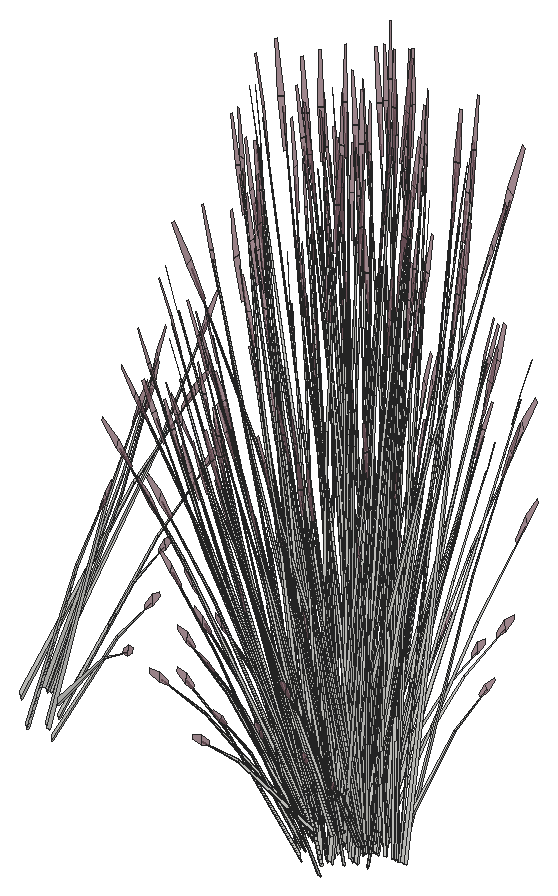
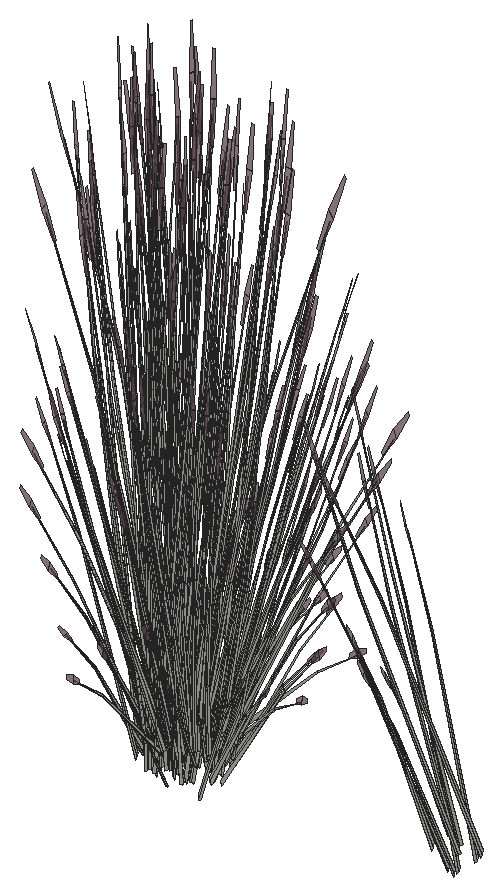
# SketchUp Ruby script. Lengths in inches.
U = 1.inch
M = Sketchup.active_model
def pt(a) = Geom::Point3d.new(a.map { |v| v * U })
def face(e, loops, mat)
  f = e.add_face(loops[0].map { |a| pt(a) })
  loops[1..].each { |l| e.add_face(l.map { |a| pt(a) }).erase! }
  f.material = f.back_material = mat if mat
  f
end
# faces: each face lists its corners as indices into pts; further lists are holes
def faces(e, pts, list, mat = nil) = list.each { |f| face(e, (f[0].is_a?(Array) ? f : [f]).map { |l| l.map { |i| pts[i] } }, mat) }
# xy, xz, yz: faces in a plane at the given z, y or x. An outline is a flat list of corners, or four numbers for a rectangle; further outlines are holes
def ring(l) = l.size == 4 ? [[l[0], l[1]], [l[2], l[1]], [l[2], l[3]], [l[0], l[3]]] : l.each_slice(2).to_a
def flat(e, list, mat, &to3) = list.each { |f| face(e, (f[0].is_a?(Array) ? f : [f]).map { |l| ring(l).map { |u, v| to3.(u, v) } }, mat) }
def xy(e, z, list, mat = nil) = flat(e, list, mat) { |x, y| [x, y, z] }
def xz(e, y, list, mat = nil) = flat(e, list, mat) { |x, z| [x, y, z] }
def yz(e, x, list, mat = nil) = flat(e, list, mat) { |y, z| [x, y, z] }
def lines(e, pts, list) = list.each { |a, b| e.add_line(pt(pts[a]), pt(pts[b])) }
# prism: a flat outline (further loops are holes) pulled along v
def prism(e, loops, v, mat = nil)
  f = face(e, loops, mat); d = Geom::Vector3d.new(v.map { |x| x * U })
  f.pushpull(f.normal.samedirection?(d) ? d.length : -d.length)
end
def box(e, o, s, mat = nil) = prism(e, [[o, [o[0] + s[0], o[1], o[2]], [o[0] + s[0], o[1] + s[1], o[2]], [o[0], o[1] + s[1], o[2]]]], [0, 0, s[2]], mat)
def at(x, y, z, deg = 0) = Geom::Transformation.translation(pt([x, y, z])) * Geom::Transformation.rotation(ORIGIN, Z_AXIS, deg.degrees)
def axes(o, x, y, z) = Geom::Transformation.new([*x, 0, *y, 0, *z, 0, *pt(o).to_a, 1])
def part(name) = M.definitions.add(name)
# library, detail: a bought-in or finely detailed component or shape, given as its bounding box
def library(name, o, s) = part(name).tap { |d| box(d.entities, o, s) }
def detail(e, o, s) = box(e.add_group.entities, o, s)
def put(e, d, t, mat = nil) = e.add_instance(d, t).tap { |i| i.material = mat if mat }
def group(e, t, mat = nil) = e.add_group.tap { |g| g.transformation = t; g.material = mat if mat }.entities
root = M.entities
M.materials.add("LightPink_Translucent").color = [144, 107, 117]
M.materials["LightPink_Translucent"].alpha = 0.75
c1 = part("blade")
p = [[2.15,0.21,22],[0,0.17,0],[0.09,0.45,0],[2.18,0.31,22],[2.29,0.31,22],[0.38,0.45,0],
  [2.48,0.24,33],[2.49,0.24,33],[2.48,0.22,33]]
faces(c1.entities,p,[[0,1,2,3],[4,5,2,3],[6,3,4,7],[8,0,3,6]])
c2 = part("seeds")
p = [[0.3,-0.1,1.38],[-0.01,-0.03,1.59],[-0.01,-0.03,0.03],[0.14,-0.07,-0.07],[0.29,-0.03,3],[0.15,0.01,3.11]]
faces(c2.entities,p,[[0,1,2,3],[1,0,4,5]],"LightPink_Translucent")
c3 = part("blade with seeds")
put(c3.entities,c1,at(0,0,0))
put(c3.entities,c2,axes([2.4,0.25,30.99],[1.5799,-0.05474,1.17369],[-0.12525,1.92788,0.29478],[-0.07173,-0.02425,1.56792]))
put(root,c3,axes([320.12,11.77,-3.41],[-0.27143,-0.0181,1.43002],[-0.27808,-0.48551,-0.30754],[0.33346,-0.13735,0.61141]))
put(root,c3,axes([320.3,13.48,-1.47],[0.63144,0.17046,-0.35414],[-0.18417,0.49731,0.4572],[0.25423,-0.0456,0.87481]))
put(root,c3,axes([319.08,14.55,-1.02],[0.75952,0.01471,-0.71045],[-0.05101,0.61953,0.08574],[0.32177,0.06538,1.00501]))
put(root,c3,axes([320.62,13.38,-4.02],[-0.48937,0.07333,1.41583],[-0.07789,-0.58369,0.08104],[0.34275,-0.08835,0.80566]))
put(root,c3,axes([321.15,13,-4.51],[-0.03971,-0.09277,1.76342],[0.27541,-0.54264,-0.26939],[0.27782,-0.00781,0.30037]))
put(root,c3,axes([321.42,15.34,-1.29],[-0.0687,-0.05349,1.77383],[0.15029,-0.57341,-0.16761],[0.27062,-0.03664,0.31391]))
put(root,c3,axes([318.58,12.86,-2.125],[-0.31515,0.01384,1.71376],[0.20907,-0.5998,0.13857],[0.44912,0.0371,0.73262]))
put(root,c3,axes([319.73,13.43,-1.02],[0.66765,-0.26986,-0.71045],[0.37208,0.55551,0.08574],[0.32259,-0.0631,1.00501]))
put(root,c3,axes([321.97,12.83,-1.28],[0.10543,-0.09307,1.74944],[-0.13495,-0.57092,-0.27667],[0.26455,-0.10825,0.14031]))
put(root,c3,axes([320.76,14.25,-3.41],[-0.18299,-0.15028,1.43002],[0.23809,-0.49714,-0.30754],[0.37023,0.06735,0.61141]))
put(root,c3,axes([344.33,12.17,-2.125],[0.31515,-0.01384,1.71376],[-0.20907,0.5998,0.13857],[-0.44912,-0.0371,0.73262]))
put(root,c3,axes([344.46,13.23,-2.125],[0.26363,-0.12925,1.71376],[0.22195,0.59723,0.13857],[-0.41388,0.13498,0.73262]))
put(root,c3,axes([343.64,14.24,-3.41],[0.26405,0.05016,1.43002],[0.17019,0.51235,-0.30754],[-0.35868,0.0959,0.61141]))
put(root,c3,axes([345.97,12.6,-2.66],[0.21597,-0.08839,1.77064],[0.07448,0.61717,0.13857],[-0.4678,0.08189,0.63284]))
put(root,c3,axes([343.65,13.02,-1.28],[-0.12407,0.07933,1.74944],[0.01055,0.57963,-0.27667],[-0.2844,0.07538,0.14031]))
put(root,c3,axes([345.27,11.61,-1.02],[-0.75952,-0.01471,-0.71045],[0.05101,-0.61953,0.08574],[-0.32177,-0.06538,1.00501]))
put(root,c3,axes([344.66,11.76,-3.41],[0.14835,0.17012,1.43002],[-0.34183,0.46242,-0.30754],[-0.351,-0.11053,0.61141]))
put(root,c3,axes([344.05,12.6875,-1.47],[-0.63144,-0.17046,-0.35414],[0.18417,-0.49731,0.4572],[-0.25423,0.0456,0.87481]))
put(root,c3,axes([344.92,11.21,-2.125],[0.28223,0.10528,1.71376],[-0.58406,0.44165,0.13857],[-0.36402,-0.19924,0.73262]))
put(root,c3,axes([342.27,13.6,-1.29],[0.09697,0.01639,1.77383],[0.29997,0.53988,-0.16761],[-0.1985,0.1417,0.31391]))
put(root,c3,axes([344.48,12.94,-1.32],[-0.20584,0.55581,-0.51099],[-0.70573,-0.19051,-0.3958],[-0.28414,0.05097,0.97773]))
put(root,c3,axes([345.02,11.74,-1.32],[-0.55171,0.40476,-0.51099],[-0.48318,-0.42758,-0.3958],[-0.28031,-0.06159,0.97773]))
put(root,c3,axes([344.13,12.91,-4.51],[0.01927,0.0963,1.76342],[-0.38846,0.5029,-0.26939],[-0.27592,-0.02535,0.30037]))
put(root,c3,axes([344.24,10.6,-1.29],[0.05633,0.06098,1.77383],[-0.27155,0.54815,-0.16761],[-0.27501,0.00397,0.31391]))
put(root,c3,axes([343.09,15.32,-3.23],[0.31665,-0.27694,1.1486],[0.12495,0.43841,0.84392],[-0.22883,0.0785,0.25299]))
put(root,c3,axes([344.87,10.24,-1.28],[-0.16348,-0.00431,1.74944],[-0.52047,0.43131,-0.27667],[-0.2777,-0.08813,0.14031]))
put(root,c3,axes([344.2,12.625,-1.27],[0.21466,-0.55714,0.48003],[0.70573,0.19051,0.3958],[-0.27753,0.03348,0.9933]))
put(root,c3,axes([344.45,12.46,-0.97],[0.38229,0.5533,-0.1216],[-0.6785,0.2719,-0.67495],[-0.28593,0.073,1.02557]))
put(root,c3,axes([345.31,11.32,-0.97],[-0.04068,0.62141,-0.1216],[-0.77029,-0.01698,-0.67495],[-0.29667,-0.04317,1.02557]))
put(root,c3,axes([344.81,11.36,-1.47],[-0.43232,-0.38257,-0.35414],[0.49364,-0.36215,0.4572],[-0.25081,-0.0551,0.87481]))
put(root,c3,axes([344.14,12.48,-1.27],[-0.27906,-0.41663,0.0643],[0.50888,-0.20393,0.50621],[-0.22432,0.04024,0.77189]))
put(root,c3,axes([345.42,13.63,-2.125],[0.18977,-0.18775,1.71376],[0.47917,0.50677,0.13857],[-0.32866,0.23079,0.73262]))
put(root,c3,axes([344.28,14.12,-1.47],[-0.66138,0.08733,-0.35414],[-0.17464,-0.49921,0.4572],[-0.18953,0.13408,0.87481]))
put(root,c3,axes([343.92,15.6,-4.51],[0.10192,0.06105,1.76342],[0.17281,0.56562,-0.26939],[-0.22588,0.12062,0.30037]))
put(root,c3,axes([343.78,12.28,-3.23],[0.48508,-0.04372,1.1486],[-0.3077,0.38525,0.84392],[-0.23971,-0.05779,0.25299]))
put(root,c3,axes([344.37,14.01,-1.27],[-0.18844,-0.56237,0.48003],[0.73919,-0.0976,0.3958],[-0.21785,0.13226,0.9933]))
put(root,c3,axes([344.75,11.21,-0.91],[0.62747,-0.45094,0.53763],[0.54116,0.47889,0.4433],[-0.29439,-0.08318,1.11249]))
put(root,c3,axes([344.22,13.9,-1.27],[-0.52161,-0.25698,0.0643],[0.30368,-0.36595,0.50621],[-0.16723,0.11831,0.77189]))
put(root,c3,axes([345.28,14.09,-2.125],[0.14147,-0.21002,1.71376],[0.59349,0.43464,0.13857],[-0.26773,0.27089,0.73262]))
put(root,c3,axes([344.72,12.63,-0.95],[0.63144,0.17046,0.35414],[-0.18417,0.49731,-0.4572],[-0.25423,0.0456,0.87481]))
put(root,c3,axes([344.83,14.18,-1.32],[0.19519,0.55794,-0.51099],[-0.73919,0.0976,-0.3958],[-0.21183,0.14986,0.97773]))
put(root,c3,axes([345.04,11.21,-1.27],[0.03826,-0.46465,0.0643],[0.57772,0.01274,0.50621],[-0.2213,-0.04862,0.77189]))
put(root,c3,axes([343.67,15.18,-1.28],[-0.01889,0.12092,1.74944],[0.53598,0.42065,-0.27667],[-0.14032,0.19892,0.14031]))
put(root,c3,axes([346.67,13.78,-3.94],[-0.79037,-0.10018,-0.62353],[0.16679,-0.61794,-0.16365],[-0.23587,-0.07488,1.37633]))
put(root,c3,axes([346.8125,10.41,-0.57],[-0.50709,0.58578,-0.13619],[-0.73436,-0.33748,-0.75594],[-0.25527,-0.1655,1.14864]))
put(root,c3,axes([345.43,11.56,-0.95],[0.43232,0.38257,0.35414],[-0.49364,0.36215,-0.4572],[-0.25081,-0.0551,0.87481]))
put(root,c3,axes([346.59,10.88,-1.02],[-0.64788,-0.29534,-0.71045],[0.46044,-0.51755,0.08574],[-0.23473,-0.17635,1.00501]))
put(root,c3,axes([346.29,10.9,-1.32],[-0.74975,0.14525,-0.51099],[-0.13115,-0.55007,-0.3958],[-0.20138,-0.15763,0.97773]))
put(root,c3,axes([345.63,14.95,-3.98],[-0.7111,-0.30552,-0.49651],[0.42504,-0.54784,0],[-0.16196,-0.06958,1.57504]))
put(root,c3,axes([345.32,10.4,-4.51],[-0.0736,0.08049,1.76342],[-0.74378,0.17355,-0.26939],[-0.17968,-0.15788,0.30037]))
put(root,c3,axes([344.48,13.78,-0.97],[0.70283,0.33692,-0.1216],[-0.40491,0.48793,-0.67495],[-0.19857,0.16961,1.02557]))
put(root,c3,axes([346.07,15.32,-3.625],[-0.47504,0.61229,0],[-0.79476,-0.34146,-0.51607],[-0.18101,-0.07777,1.63711]))
put(root,c3,axes([343.32,15.24,-0.35],[0.67048,0.16311,-0.06488],[-0.20625,0.50201,-0.29416],[-0.10966,0.07622,0.97024]))
put(root,c3,axes([344.82,13.83,-0.95],[0.66138,-0.08733,0.35414],[0.17464,0.49921,-0.4572],[-0.18953,0.13408,0.87481]))
put(root,c3,axes([345.2,16.2,-3.41],[0.23977,-0.09639,1.43002],[0.59198,0.29065,-0.30754],[-0.1762,0.25149,0.61141]))
put(root,c3,axes([344.86,10.71,-3.87],[-0.21918,0.49894,-0.03893],[-0.6746,-0.15348,-0.17649],[-0.10242,-0.08161,0.58215]))
put(root,c3,axes([346.62,9.02,-1.29],[-0.01417,0.07324,1.77383],[-0.6991,0.2658,-0.16761],[-0.20573,-0.13587,0.31391]))
put(root,c3,axes([345.87,10.08,-3.41],[-0.04601,0.19989,1.43002],[-0.67263,0.16733,-0.30754],[-0.15723,-0.25836,0.61141]))
put(root,c3,axes([346.09,10.6,-2.125],[0.17368,0.19618,1.71376],[-0.80256,0.16516,0.13857],[-0.18139,-0.30799,0.73262]))
put(root,c3,axes([347.57,13.87,-3.33],[-0.76714,0.40567,-0.29095],[-0.51013,-0.57321,-0.50002],[-0.18927,-0.05821,1.59708]))
put(root,c3,axes([345.45,15.15,-1.27],[-0.54105,-0.41691,0.48003],[0.57458,-0.35956,0.3958],[-0.0998,0.1956,0.9933]))
put(root,c3,axes([346.37,10.49,-1.47],[-0.11735,-0.49217,-0.35414],[0.67083,-0.12996,0.4572],[-0.18018,-0.14104,0.87481]))
put(root,c3,axes([344.5,12.99,-3.625],[-0.95008,0,0],[0,-0.68292,-0.51607],[0,-0.15554,1.63711]))
put(root,c3,axes([345.83,14.72,-3.97],[-0.17848,-0.53243,-0.30978],[0.70886,-0.15119,0.30978],[-0.1429,-0.0614,1.38974]))
put(root,c3,axes([345.25,15.11,-1.27],[-0.62439,-0.02847,0.0643],[0.01712,-0.42991,0.50621],[-0.06534,0.16468,0.77189]))
put(root,c3,axes([345.45,15.28,-1.47],[-0.5141,0.32171,-0.35414],[-0.48666,-0.36734,0.4572],[-0.07405,0.18664,0.87481]))
put(root,c3,axes([348.08,14.3125,-3.94],[-0.51177,0.45928,-0.62353],[-0.63575,-0.41646,-0.16365],[-0.20507,0.11457,1.37633]))
put(root,c3,axes([346.76,10.89,-0.95],[0.11735,0.49217,0.35414],[-0.67083,0.12996,-0.4572],[-0.18018,-0.14104,0.87481]))
put(root,c3,axes([343.61,16.42,-1.29],[0.0862,-0.03689,1.77383],[0.71245,0.24539,-0.16761],[-0.01674,0.20431,0.31391]))
put(root,c3,axes([345.23,12.81,-3.67],[-0.70674,0.51372,0.30756],[-0.70717,-0.50832,-0.36492],[-0.02468,-0.14589,1.64885]))
put(root,c3,axes([348.14,14.22,-2.67],[0.65659,0.2464,1.51261],[-0.64324,0.53082,0.59816],[-0.28812,-0.31461,1.26806]))
put(root,c3,axes([345.64,9.76,-3.23],[0.39634,0.21267,1.1486],[-0.57721,0.12784,0.84392],[-0.1235,-0.16344,0.25299]))
put(root,c3,axes([348.43,14.05,-3.54],[-0.74193,-0.49181,-0.25192],[0.6243,-0.55226,0.5513],[-0.19979,0.05753,1.68216]))
put(root,c3,axes([347.08,13.58,-3.79],[-0.45644,-0.51287,-0.44739],[0.69137,-0.36116,0.21531],[-0.14771,-0.06346,1.43643]))
put(root,c3,axes([345.79,14.9375,-0.66],[-0.01977,0.56521,-0.7886],[-0.83252,-0.03796,0.09517],[-0.08786,0.23945,1.11556]))
put(root,c3,axes([345.77,16.53,-3.23],[-0.01966,-0.36332,1.1486],[0.49135,0.25914,0.84392],[-0.09663,0.17317,0.25299]))
put(root,c3,axes([346.46,10.31,-0.91],[0.84639,-0.15705,0.53763],[0.14689,0.61608,0.4433],[-0.19906,-0.18157,1.11249]))
put(root,c3,axes([348.05,13.95,-3.79],[-0.82508,0.03772,-0.44739],[-0.07462,-0.62614,0.21531],[-0.14771,0.06346,1.43643]))
put(root,c3,axes([346.66,10.45,-1.27],[0.34533,-0.38816,0.0643],[0.49176,0.22599,0.50621],[-0.15898,-0.12445,0.77189]))
put(root,c3,axes([346.48,15,-3.52],[0.7111,0.30552,0.49651],[-0.42504,0.54784,0],[-0.16196,-0.06958,1.57504]))
put(root,c3,axes([345.51,15.73,-2.64],[0.01669,-0.31544,1.54345],[0.75083,0.16661,0.21329],[-0.06506,0.33618,0.72882]))
put(root,c3,axes([347.15,13.875,-3.5625],[0.20138,-0.72405,-0.23429],[0.95485,0.12621,0.51271],[-0.16685,-0.09999,1.5644]))
put(root,c3,axes([347.49,14.05,-3.38],[-0.14658,0.54532,0.1448],[-0.71613,-0.09466,-0.41347],[-0.13033,-0.05599,1.26744]))
put(root,c3,axes([347.41,9.3,-1.28],[-0.11621,-0.08567,1.74944],[-0.77555,0.05431,-0.27667],[-0.12378,-0.20491,0.14031]))
put(root,c3,axes([348.92,15.57,-3.98],[-0.7111,0.30552,-0.49651],[-0.42504,-0.54784,0],[-0.16196,0.06958,1.57504]))
put(root,c3,axes([344.71,12.52,-3.98],[0,-0.61104,-0.49651],[0.85008,0,0],[0,-0.13917,1.57504]))
put(root,c3,axes([345.07,13.09,-3.52],[0,0.61104,0.49651],[-0.85008,0,0],[0,-0.13917,1.57504]))
put(root,c3,axes([348.97,15.4,-3.81],[-0.46912,-0.61443,-0.05142],[0.79476,-0.34146,0.51607],[-0.19584,0.0585,1.6363]))
put(root,c3,axes([345.96,15.125,-1],[0.54391,0.41056,-0.5672],[-0.57458,0.35956,-0.43934],[-0.08276,0.2086,1.08528]))
put(root,c3,axes([348.75,15.32,-3.97],[-0.70886,-0.15119,-0.30978],[0.17848,-0.53243,0.30978],[-0.1429,0.0614,1.38974]))
put(root,c3,axes([345.71,14.82,-0.95],[0.5141,-0.32171,0.35414],[0.48666,0.36734,-0.4572],[-0.07405,0.18664,0.87481]))
put(root,c3,axes([346.93,13.23,-3.33],[-0.85568,-0.29155,-0.29095],[0.41201,-0.61537,-0.50002],[-0.02689,-0.15109,1.59708]))
put(root,c3,axes([349.16,13.05,-3.16],[-0.02076,-0.57531,1.41272],[0.93937,0.14913,0.59816],[-0.22217,0.31481,1.3335]))
put(root,c3,axes([345.39,14.91,-0.6],[0.83505,0.03027,-0.13498],[-0.02282,0.57322,-0.74919],[-0.05801,0.22077,1.13838]))
put(root,c3,axes([345.37,15.74,-3.18],[0.69024,-0.1082,0.06507],[0.15868,0.43593,-0.86304],[-0.04376,0.22067,0.7736]))
put(root,c3,axes([348.63,13.78,-3.33],[0.08854,0.69723,-0.29095],[-0.92215,0.04216,-0.50002],[-0.16238,0.09287,1.59708]))
put(root,c3,axes([346.55,12.61,-3.9],[-0.31203,-0.62659,-0.69835],[0.89884,-0.22566,-0.18329],[-0.03449,-0.21218,1.54149]))
put(root,c3,axes([348.59,10.62,-0.97],[-0.74352,0.28449,-0.1216],[-0.36538,-0.50492,-0.67495],[-0.0981,-0.21277,1.02557]))
put(root,c3,axes([347.95,10.64,-1.32],[-0.7469,-0.15318,-0.51099],[0.25601,-0.52518,-0.3958],[-0.06849,-0.21144,0.97773]))
put(root,c3,axes([346.58,14.54,-2.125],[-0.0186,-0.23452,1.71376],[0.80601,0.15558,0.13857],[-0.04985,0.33422,0.73262]))
put(root,c3,axes([345.07,12.54,-3.97],[0.53038,-0.38124,-0.30978],[0.53038,0.38124,0.30978],[0,-0.1228,1.38974]))
put(root,c3,axes([347.47,10.07,-3.87],[-0.52505,0.35054,-0.03893],[-0.48109,-0.38392,-0.17649],[-0.03387,-0.10878,0.58215]))
put(root,c3,axes([347.26,13.53,-3.64],[0.96033,0.12874,0.45755],[-0.19544,0.7271,0.17955],[-0.14034,-0.07021,1.58856]))
put(root,c3,axes([347.01,13.4,-3.28],[-0.36864,0.55059,0.44739],[-0.76598,-0.26498,-0.21531],[0,-0.12692,1.43643]))
put(root,c3,axes([348.23,10.74,-1.02],[-0.36264,-0.49684,-0.71045],[0.74649,-0.27689,0.08574],[-0.0848,-0.24006,1.00501]))
put(root,c3,axes([346.74,14.6875,-3.53],[0.81646,-0.16218,0.17642],[0.20161,0.60355,0.35086],[-0.07282,-0.08794,1.60407]))
put(root,c3,axes([347.79,14.78,-3.8],[-0.76598,-0.27433,0],[0.36864,-0.57001,0],[0,0,1.62707]))
put(root,c3,axes([348.37,10.82,-0.95],[-0.22906,0.4699,0.35414],[-0.66828,-0.13705,-0.4572],[-0.06128,-0.18919,0.87481]))
put(root,c3,axes([349.57,15.47,-3.625],[0.47504,0.61229,0],[-0.79476,0.34146,-0.51607],[-0.18101,0.07777,1.63711]))
put(root,c3,axes([347.15,15.73,-0.9375],[-0.74868,-0.15974,0.53283],[0.25601,-0.52518,0.43934],[0.04499,0.20653,1.10256]))
put(root,c3,axes([346.95,15.77,-1.27],[-0.55987,0.20767,0.0643],[-0.27403,-0.37869,0.50621],[0.05407,0.16693,0.77189]))
put(root,c3,axes([349.17,14.72,-3.53],[0.21949,-0.60727,0.17642],[0.8032,0.17185,0.35086],[-0.13875,0.00296,1.60407]))
put(root,c3,axes([348.8,13.92,-3.38],[0.56134,0.36712,0.1448],[-0.46823,0.41419,-0.41347],[-0.13033,0.05599,1.26744]))
put(root,c3,axes([348.6,13.46,-3.7],[-0.70674,-0.52593,-0.06131],[0.70717,-0.52625,0],[-0.02468,-0.01837,1.75571]))
put(root,c3,axes([348.79,13.65,-3.28],[0.82508,-0.03772,0.44739],[0.07462,0.62614,-0.21531],[-0.14771,0.06346,1.43643]))
put(root,c3,axes([348.99,15.09,-3.67],[0.95122,0.19861,0.30756],[-0.23797,0.7099,-0.36492],[-0.15744,0.08885,1.64885]))
put(root,c3,axes([347.6,9.64,-4.51],[-0.12744,0.02202,1.76342],[-0.70477,-0.24781,-0.26939],[0.01183,-0.2067,0.30037]))
put(root,c3,axes([349.4,15.05,-3.52],[0.7111,-0.30552,0.49651],[0.42504,0.54784,0],[-0.16196,0.06958,1.57504]))
put(root,c3,axes([348.29,10.32,-1.47],[0.22906,-0.4699,-0.35414],[0.66828,0.13705,0.4572],[-0.06128,-0.18919,0.87481]))
put(root,c3,axes([347.18,12.86,-3.64],[0.33034,0.68327,0.45755],[-0.94388,0.2376,0.17955],[0.01154,-0.12555,1.58856]))
put(root,c3,axes([347.02,12.77,-3.79],[0.36864,-0.55059,-0.44739],[0.76598,0.26498,0.21531],[0,-0.12692,1.43643]))
put(root,c3,axes([347.97,14.55,-3.8],[-0.24791,-0.5268,0],[0.70791,-0.18448,0],[0,0,1.54371]))
put(root,c3,axes([347.07,15.66,-4.51],[0.12297,-0.03325,1.76342],[0.73967,0.18301,-0.26939],[0.02163,0.20626,0.30037]))
put(root,c3,axes([347.23,15.84,-1.47],[-0.22906,0.4699,-0.35414],[-0.66828,-0.13705,0.4572],[0.06128,0.18919,0.87481]))
put(root,c3,axes([348.97,13.51,-3.79],[-0.36864,0.55059,-0.44739],[-0.76598,-0.26498,0.21531],[0,0.12692,1.43643]))
put(root,c3,axes([348.58,10.39,-1.27],[0.55987,-0.20767,0.0643],[0.27403,0.37869,0.50621],[-0.05407,-0.16693,0.77189]))
put(root,c3,axes([346.76,16.68,-1.28],[0.09631,0.0984,1.74944],[0.77725,0.03866,-0.27667],[0.07816,0.217,0.14031]))
put(root,c3,axes([350.43,13.17,-3.53],[-0.59697,-0.44509,0.17642],[0.60159,-0.4317,0.35086],[-0.06593,0.0909,1.60407]))
put(root,c3,axes([348.36,12.92,-3.79],[0,-0.70701,0],[0.95008,0,0],[0,0,1.79456]))
put(root,c3,axes([348.38,10.43,-1.27],[0.74868,0.15974,0.48003],[-0.25601,0.52518,0.3958],[-0.04499,-0.20653,0.9933]))
put(root,c3,axes([347.48,13.04,-3.57],[0.8561,0.29616,0.24065],[-0.41201,0.61537,0.50002],[0,-0.14185,1.60543]))
put(root,c3,axes([348.84,13.2,-3.71],[0,0.70667,-0.05637],[-0.95008,0,0],[0,0.02221,1.79368]))
put(root,c3,axes([347.2,12.63,-3.28],[-0.82508,0.03772,0.44739],[-0.07462,-0.62614,-0.21531],[0.14771,-0.06346,1.43643]))
put(root,c3,axes([347.16,15.35,-0.95],[0.22906,-0.4699,0.35414],[0.66828,0.13705,-0.4572],[0.06128,0.18919,0.87481]))
put(root,c3,axes([346.82,11.56,-3.53],[-0.21949,0.60727,0.17642],[-0.8032,-0.17185,0.35086],[0.13875,-0.00296,1.60407]))
put(root,c3,axes([348.39,14.57,-3.71],[0.33034,0.70197,-0.06012],[-0.94388,0.24598,0],[0.01154,0.02451,1.72173]))
put(root,c3,axes([346.43,10.81,-3.625],[-0.47504,-0.61229,0],[0.79476,-0.34146,-0.51607],[0.18101,-0.07777,1.63711]))
put(root,c3,axes([347.3,15.42,-1.02],[0.36264,0.49684,-0.71045],[-0.74649,0.27689,0.08574],[0.0848,0.24006,1.00501]))
put(root,c3,axes([351.11,13.64,-3.8],[-0.94962,-0.00489,-0.04976],[0,-0.68292,0.49943],[-0.02984,0.15546,1.58352]))
put(root,c3,axes([349.25,11.59,-3.53],[-0.81646,0.16218,0.17642],[-0.20161,-0.60355,0.35086],[0.07282,0.08794,1.60407]))
put(root,c3,axes([348.42,9.33,-3.23],[0.09747,0.35631,1.1486],[-0.54071,-0.19735,0.84392],[0.05818,-0.18244,0.25299]))
put(root,c3,axes([348.06,17.03,-0.35],[0.52505,-0.35054,-0.06488],[0.48109,0.38392,-0.29416],[0.03387,0.10878,0.97024]))
put(root,c3,axes([347.91,12.47,-3.64],[-0.62999,0.55453,0.45755],[-0.74845,-0.4895,0.17955],[0.15188,-0.05534,1.58856]))
put(root,c3,axes([348.99,13.34,-3.79],[0.53038,0.39469,0],[-0.53038,0.39469,0],[0,0,1.69266]))
put(root,c3,axes([348.98,12.88,-3.28],[0.36864,-0.55059,0.44739],[0.76598,0.26498,-0.21531],[0,0.12692,1.43643]))
put(root,c3,axes([348.66,14.8,-3.8],[0.76598,0.27433,0],[-0.36864,0.57001,0],[0,0,1.74954]))
put(root,c3,axes([347.57,15.52,-1.32],[0.7469,0.15318,-0.51099],[-0.25601,0.52518,-0.3958],[0.06849,0.21144,0.97773]))
put(root,c3,axes([346.93,15.55,-0.97],[0.74352,-0.28449,-0.1216],[0.36538,0.50492,-0.67495],[0.0981,0.21277,1.02557]))
put(root,c3,axes([348.73,12.75,-3.62],[-0.96033,-0.12874,0.49198],[0.19544,-0.7271,0.19306],[0.14034,0.07021,1.70813]))
put(root,c3,axes([350.73,9.91,-1.29],[-0.07716,0.04667,1.77383],[-0.75601,-0.15746,-0.16761],[-0.02737,-0.20368,0.31391]))
put(root,c3,axes([350.14,11.26,-0.97],[-0.83505,-0.03027,-0.1216],[0.02282,-0.57322,-0.67495],[0.05801,-0.22077,1.02557]))
put(root,c3,axes([350.92,13.74,-3.97],[-0.53038,0.38124,-0.30978],[-0.53038,-0.38124,0.30978],[0,0.1228,1.38974]))
put(root,c3,axes([349.4,13.67,-3.91],[0.2786,0.55945,-0.69212],[-0.80253,0.20149,-0.18165],[0.03079,0.18945,1.52773]))
put(root,c3,axes([349.01,13.07,-3.79],[0.85008,0,0],[0,0.63259,0],[0,0,1.78407]))
put(root,c3,axes([349.81,11.35,-0.95],[-0.5141,0.32171,0.35414],[-0.48666,-0.36734,-0.4572],[0.07405,-0.18664,0.87481]))
put(root,c3,axes([348.19,12.375,-3.28],[-0.45644,-0.51287,0.44739],[0.69137,-0.36116,-0.21531],[0.14771,0.06346,1.43643]))
put(root,c3,axes([347.36,12.5,-3.33],[-0.08854,-0.69723,-0.29095],[0.92215,-0.04216,-0.50002],[0.16238,-0.09287,1.59708]))
put(root,c3,axes([349.3,13.01,-3.38],[0.70791,-0.1782,0.1448],[0.24791,0.50885,-0.41347],[0,0.11199,1.26744]))
put(root,c3,axes([349.57,11.04,-1.32],[-0.54391,-0.41056,-0.51099],[0.57458,-0.35956,-0.3958],[0.08276,-0.2086,0.97773]))
put(root,c3,axes([349.06,13.05,-3.33],[0.85568,0.29155,-0.29095],[-0.41201,0.61537,-0.50002],[0.02689,0.15109,1.59708]))
put(root,c3,axes([347.24,10.95,-3.97],[0.70886,0.15119,-0.30978],[-0.17848,0.53243,0.30978],[0.1429,-0.0614,1.38974]))
put(root,c3,axes([349.21,10.3125,-3.41],[-0.21597,0.12368,1.43002],[-0.64681,-0.21647,-0.30754],[0.1199,-0.26922,0.61141]))
put(root,c3,axes([350.92,13.19,-3.52],[0,-0.61104,0.49651],[0.85008,0,0],[0,0.13917,1.57504]))
put(root,c3,axes([351.28,13.76,-3.98],[0,0.61104,-0.49651],[-0.85008,0,0],[0,0.13917,1.57504]))
put(root,c3,axes([349.01,15.61,-1.27],[-0.75571,0.14023,0.48003],[-0.13115,-0.55007,0.3958],[0.17773,0.16212,0.9933]))
put(root,c3,axes([347.07,10.71,-3.98],[0.7111,-0.30552,-0.49651],[0.42504,0.54784,0],[0.16196,-0.06958,1.57504]))
put(root,c3,axes([348.87,15.72,-1.27],[-0.34533,0.38816,0.0643],[-0.49176,-0.22599,0.50621],[0.15898,0.12445,0.77189]))
put(root,c3,axes([347.99,14.4375,-2.125],[-0.17368,-0.19618,1.71376],[0.80256,-0.16516,0.13857],[0.18139,0.30799,0.73262]))
put(root,c3,axes([348.5,12.23,-3.38],[0.14658,-0.54532,0.1448],[0.71613,0.09466,-0.41347],[0.13033,0.05599,1.26744]))
put(root,c3,axes([349.52,11.28,-3.52],[-0.7111,-0.30552,0.49651],[0.42504,-0.54784,0],[0.16196,0.06958,1.57504]))
put(root,c3,axes([349.74,11.23,-1.02],[0.01977,-0.56521,-0.71045],[0.83252,0.03796,0.08574],[0.08786,-0.23945,1.00501]))
put(root,c3,axes([348.9,14.47,-3.82],[0.79769,-0.20732,-0.19198],[0.2803,0.59721,0.00008],[0.08805,-0.02292,1.73897]))
put(root,c3,axes([348.76,15.27,-0.95],[-0.11735,-0.49217,0.35414],[0.67083,-0.12996,-0.4572],[0.18018,0.14104,0.87481]))
put(root,c3,axes([348.91,12.7,-3.79],[0.45644,0.51287,-0.44739],[-0.69137,0.36116,0.21531],[0.14771,0.06346,1.43643]))
put(root,c3,axes([349.21,12.44,-1.53],[-0.65655,-0.31748,1.38283],[0.69326,-0.49431,0.59665],[0.21183,0.29789,1.33663]))
put(root,c3,axes([350.08,10.89,-1.47],[0.5141,-0.32171,-0.35414],[0.48666,0.36734,0.4572],[0.07405,-0.18664,0.87481]))
put(root,c3,axes([348.11,15.96,-1.29],[0.00225,-0.07398,1.77383],[0.65113,-0.32638,-0.16761],[0.22617,0.1165,0.31391]))
put(root,c3,axes([350.28,11.05,-1.27],[0.62439,0.02847,0.0643],[-0.01712,0.42991,0.50621],[0.06534,-0.16468,0.77189]))
put(root,c3,axes([350.2,15.02,-3.23],[-0.4278,-0.1757,1.1486],[0.5524,-0.17852,0.84392],[0.14899,0.15122,0.25299]))
put(root,c3,axes([348.68,14.84,-3.41],[0.01341,-0.20255,1.43002],[0.64074,-0.22625,-0.30754],[0.1978,0.24243,0.61141]))
put(root,c3,axes([350.9,10.35,-1.28],[-0.00733,-0.12161,1.74944],[-0.61946,-0.35147,-0.27667],[0.09577,-0.21306,0.14031]))
put(root,c3,axes([347.91,11.97,-3.94],[0.51177,-0.45928,-0.62353],[0.63575,0.41646,-0.16365],[0.20507,-0.11457,1.37633]))
put(root,c3,axes([350.08,11.01,-1.27],[0.54105,0.41691,0.48003],[-0.57458,0.35956,0.3958],[0.0998,-0.1956,0.9933]))
put(root,c3,axes([350.16,11.56,-3.97],[0.17848,0.53243,-0.30978],[-0.70886,0.15119,0.30978],[0.1429,0.0614,1.38974]))
put(root,c3,axes([351.49,13.29,-3.625],[0.95008,0,0],[0,0.68292,-0.51607],[0,0.15554,1.63711]))
put(root,c3,axes([348.42,12.41,-3.33],[0.76714,-0.40567,-0.29095],[0.51013,0.57321,-0.50002],[0.18927,0.05821,1.59708]))
put(root,c3,axes([350.27,15.82,-3.33],[-0.48723,-0.01916,1.0506],[0.32177,-0.40701,0.58006],[0.19248,0.1446,0.8241]))
put(root,c3,axes([350.7,12.34,-0.95],[-0.66138,0.08733,0.35414],[-0.17464,-0.49921,-0.4572],[0.18953,-0.13408,0.87481]))
put(root,c3,axes([348.8,10.94,-2.125],[-0.14147,0.21002,1.71376],[-0.59349,-0.43464,0.13857],[0.26773,-0.27089,0.73262]))
put(root,c3,axes([348.7,15.53,-0.97],[0.45276,-0.52302,-0.1216],[0.65568,0.30132,-0.67495],[0.22792,0.14777,1.02557]))
put(root,c3,axes([346.49,12.05,-4.41],[-0.74787,0.24464,1.28929],[-0.23804,-0.70192,0.50096],[0.45924,0.01168,1.46642]))
